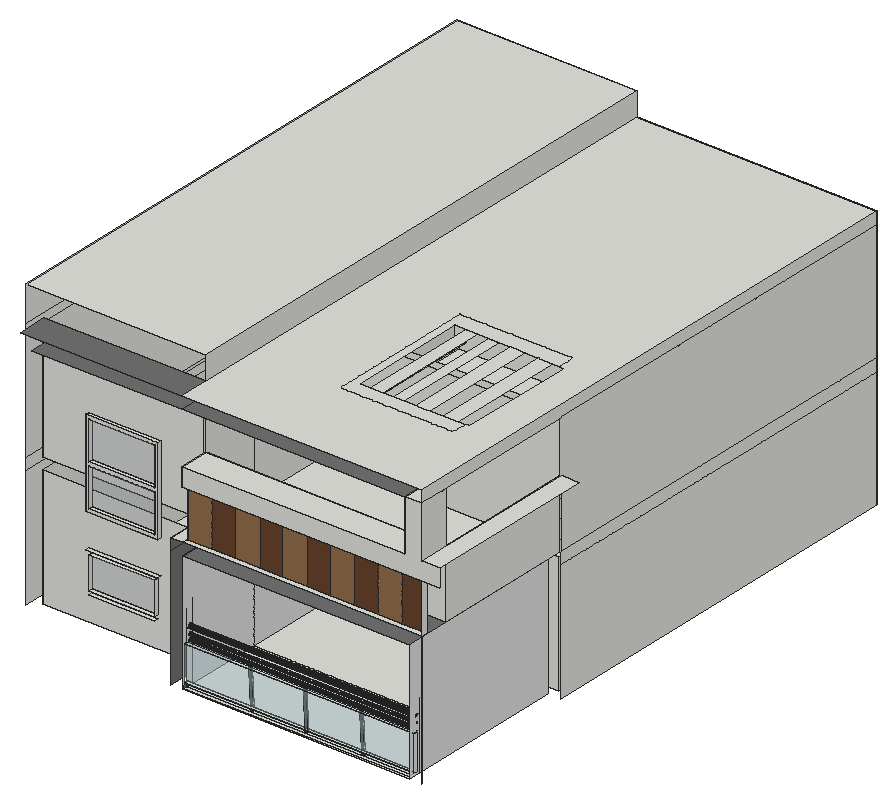
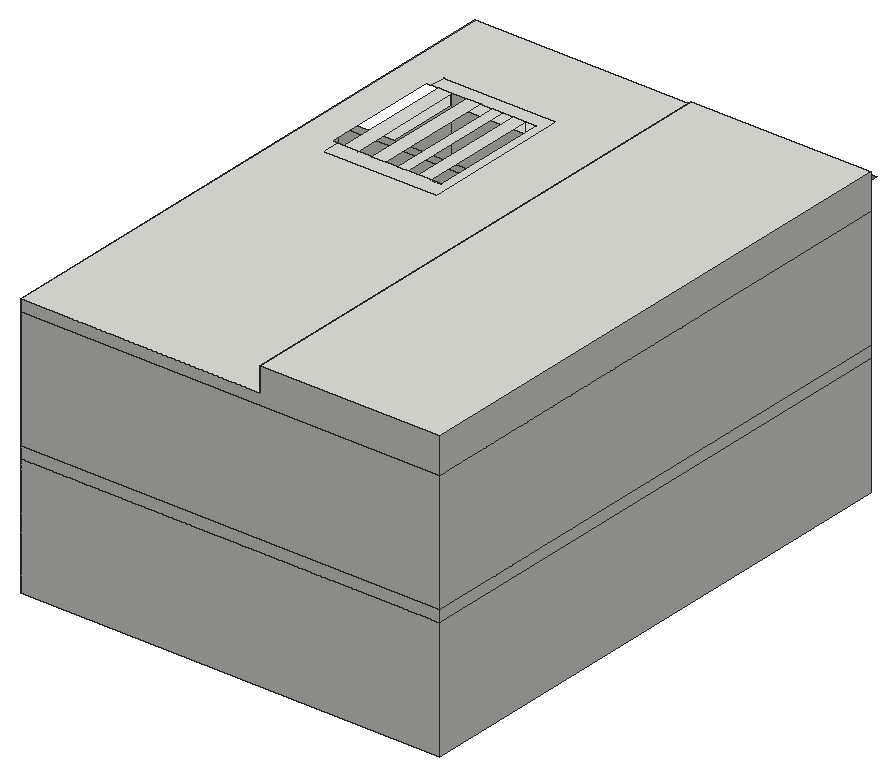
# SketchUp Ruby script. Lengths in inches.
U = 1.inch
M = Sketchup.active_model
def pt(a) = Geom::Point3d.new(a.map { |v| v * U })
def face(e, loops, mat)
  f = e.add_face(loops[0].map { |a| pt(a) })
  loops[1..].each { |l| e.add_face(l.map { |a| pt(a) }).erase! }
  f.material = f.back_material = mat if mat
  f
end
# faces: each face lists its corners as indices into pts; further lists are holes
def faces(e, pts, list, mat = nil) = list.each { |f| face(e, (f[0].is_a?(Array) ? f : [f]).map { |l| l.map { |i| pts[i] } }, mat) }
# xy, xz, yz: faces in a plane at the given z, y or x. An outline is a flat list of corners, or four numbers for a rectangle; further outlines are holes
def ring(l) = l.size == 4 ? [[l[0], l[1]], [l[2], l[1]], [l[2], l[3]], [l[0], l[3]]] : l.each_slice(2).to_a
def flat(e, list, mat, &to3) = list.each { |f| face(e, (f[0].is_a?(Array) ? f : [f]).map { |l| ring(l).map { |u, v| to3.(u, v) } }, mat) }
def xy(e, z, list, mat = nil) = flat(e, list, mat) { |x, y| [x, y, z] }
def xz(e, y, list, mat = nil) = flat(e, list, mat) { |x, z| [x, y, z] }
def yz(e, x, list, mat = nil) = flat(e, list, mat) { |y, z| [x, y, z] }
def lines(e, pts, list) = list.each { |a, b| e.add_line(pt(pts[a]), pt(pts[b])) }
# prism: a flat outline (further loops are holes) pulled along v
def prism(e, loops, v, mat = nil)
  f = face(e, loops, mat); d = Geom::Vector3d.new(v.map { |x| x * U })
  f.pushpull(f.normal.samedirection?(d) ? d.length : -d.length)
end
def box(e, o, s, mat = nil) = prism(e, [[o, [o[0] + s[0], o[1], o[2]], [o[0] + s[0], o[1] + s[1], o[2]], [o[0], o[1] + s[1], o[2]]]], [0, 0, s[2]], mat)
def at(x, y, z, deg = 0) = Geom::Transformation.translation(pt([x, y, z])) * Geom::Transformation.rotation(ORIGIN, Z_AXIS, deg.degrees)
def axes(o, x, y, z) = Geom::Transformation.new([*x, 0, *y, 0, *z, 0, *pt(o).to_a, 1])
def part(name) = M.definitions.add(name)
# library, detail: a bought-in or finely detailed component or shape, given as its bounding box
def library(name, o, s) = part(name).tap { |d| box(d.entities, o, s) }
def detail(e, o, s) = box(e.add_group.entities, o, s)
def put(e, d, t, mat = nil) = e.add_instance(d, t).tap { |i| i.material = mat if mat }
def group(e, t, mat = nil) = e.add_group.tap { |g| g.transformation = t; g.material = mat if mat }.entities
root = M.entities
M.materials.add("Glass_Basic_01").color = [161, 173, 186]
M.materials["Glass_Basic_01"].alpha = 0.25
M.materials.add("Glass_Safety_01").color = [204, 235, 244]
M.materials["Glass_Safety_01"].alpha = 0.25
M.materials.add("M00_Soft_Cloud").color = [255, 255, 255]
M.materials.add("M01_Silver_Fog").color = [224, 224, 224]
M.materials.add("M05_Graphite_Haze").color = [114, 114, 114]
M.materials.add("Metal_06_1K").color = [238, 236, 231]
M.materials.add("Wood_Floor_01_1K").color = [146, 111, 76]
M.materials.add("Wood_Veneer_15_1K").color = [103, 69, 45]
M.materials.add("[Translucent Glass Gray]").color = [132, 132, 132]
M.materials["[Translucent Glass Gray]"].alpha = 0.25
M.materials.add("[Wood Veneer 01]").color = [120, 70, 37]
c1 = part("Group\#8")
xy(c1.entities,0,[[0,0,19.69,1.18]],"[Wood Veneer 01]")
xy(c1.entities,2.76,[[2.76,0,16.93,1.18]],"[Wood Veneer 01]")
xy(c1.entities,60.24,[[2.76,0,16.93,1.18]],"[Wood Veneer 01]")
xy(c1.entities,62.99,[[0,0,19.69,1.18]],"[Wood Veneer 01]")
xz(c1.entities,0,[[2.76,2.76,16.93,60.24]],"[Translucent Glass Gray]")
xz(c1.entities,0,[[[0,0,19.69,62.99],[2.76,2.76,16.93,60.24]]],"[Wood Veneer 01]")
xz(c1.entities,1.18,[[[0,0,19.69,62.99],[2.76,2.76,16.93,60.24]]],"[Wood Veneer 01]")
yz(c1.entities,0,[[0,0,1.18,62.99]],"[Wood Veneer 01]")
yz(c1.entities,2.76,[[0,2.76,1.18,60.24]],"[Wood Veneer 01]")
yz(c1.entities,16.93,[[0,2.76,1.18,60.24]],"[Wood Veneer 01]")
yz(c1.entities,19.69,[[0,0,1.18,62.99]],"[Wood Veneer 01]")
c2 = part("pintu 2")
put(c2.entities,c1,at(-19.69,0,1.97))
g1 = group(c2.entities,at(-21.65,0,0))
prism(g1,[[[0,0,66.93],[0,0,0],[45.28,0,0],[45.28,0,66.93]],[[43.31,0,1.97],[23.62,0,1.97],[23.62,0,64.96],[43.31,0,64.96]],[[21.65,0,64.96],[21.65,0,1.97],[1.97,0,1.97],[1.97,0,64.96]]],[0,5.91,0],"[Wood Veneer 01]")
put(c2.entities,c1,at(1.97,0,1.97))
c3 = library("CLASSIC-BRASS_CHAUTAUQUA_LEVER-HARDWARE",[7.77,-2.58,0],[5.5,6.97,4.76])
xy(root,288,[[271.502,48.443,499.502,49.99],[271.502,49.99,499.502,53.035],[[271.502,53.035,499.502,59.828],[447.56,55.172,447.248,55.213,446.958,55.333,446.709,55.525,446.517,55.774,446.397,56.064,446.356,56.375,446.397,56.687,446.517,56.977,446.709,57.226,446.749,57.258,446.958,57.418,447.248,57.538,447.56,57.579,447.871,57.538,448.161,57.418,448.411,57.226,448.602,56.977,448.722,56.687,448.763,56.375,448.722,56.064,448.602,55.774,448.411,55.525,448.37,55.493,448.161,55.333,447.871,55.213],[334.673,55.172,334.361,55.213,334.071,55.333,333.822,55.525,333.63,55.774,333.51,56.064,333.469,56.375,333.51,56.687,333.63,56.977,333.822,57.226,333.897,57.284,334.071,57.418,334.361,57.538,334.673,57.579,334.984,57.538,335.274,57.418,335.523,57.226,335.715,56.977,335.835,56.687,335.876,56.375,335.835,56.064,335.715,55.774,335.523,55.525,335.448,55.467,335.274,55.333,334.984,55.213],[389.494,55.172,389.183,55.213,388.892,55.333,388.643,55.525,388.452,55.774,388.332,56.064,388.291,56.375,388.332,56.687,388.452,56.977,388.643,57.226,388.719,57.284,388.892,57.418,389.183,57.538,389.494,57.579,389.806,57.538,390.096,57.418,390.345,57.226,390.536,56.977,390.657,56.687,390.698,56.375,390.657,56.064,390.536,55.774,390.345,55.525,390.27,55.467,390.096,55.333,389.806,55.213]],[271.502,59.828,499.502,137.443],[100.502,86.443,262.502,86.443,262.502,230.443,310.876,230.443,310.876,233.831,310.201,233.831,310.201,237.474,307.502,237.474,307.502,238.931,310.876,238.931,310.876,233.831,311.213,233.831,311.213,237.474,364.86,237.474,364.86,238.931,368.234,238.931,368.234,237.474,365.534,237.474,365.534,233.831,364.86,233.831,364.86,230.443,502.502,230.443,502.502,608.443,100.502,608.443],
  [271.502,137.443,499.502,137.443,499.502,221.443,364.86,221.443,364.86,222.901,364.522,222.901,364.522,230.443,311.213,230.443,311.213,222.901,310.876,222.901,310.876,221.443,271.502,221.443],[307.502,221.443,310.876,222.901],[364.86,221.443,367.502,222.901],[367.502,221.443,368.234,222.901],[307.502,222.901,310.876,230.443],
  [310.876,222.901,311.213,230.443],[364.522,222.901,364.86,230.443],[364.86,222.901,367.502,230.443],[310.876,230.443,311.213,230.443,311.213,233.831,310.876,233.831,310.876,237.474,310.201,237.474,310.201,233.831,310.876,233.831],[311.213,230.443,364.522,233.831],
  [364.522,230.443,364.86,231.645],[364.522,231.645,364.86,231.645,364.86,233.831,365.197,233.831,365.197,237.474,364.86,237.474,364.86,233.831,364.522,233.831],[311.213,233.831,364.86,237.474],[365.197,233.831,365.534,237.474],[307.502,237.474,310.876,238.931],
  [364.86,237.474,368.234,238.931]])
xy(root,291.818,[[324.034,233.831,324.709,234.559],[324.034,236.745,324.709,237.474]])
xy(root,293.1875,[[271.502,49.99,502.148,53.035]])
xy(root,306.378,[[410.693,221.443,458.693,230.443]],"M00_Soft_Cloud")
xy(root,322.044,[[157.502,73.443,223.502,77.443]])
xy(root,325.044,[[157.502,73.443,223.502,77.443]])
xy(root,328.294,[[271.502,49.99,502.148,53.035]],"Glass_Safety_01")
xy(root,358.044,[[157.502,73.443,223.502,77.443]])
xy(root,361.044,[[154.502,73.443,226.502,77.443]])
xy(root,366.273,[[324.034,233.831,324.709,234.559],[324.034,236.745,324.709,237.474]])
xy(root,369.9,[[311.213,222.901,364.522,233.831]])
xy(root,370.091,[[310.876,221.443,364.86,222.901],[364.522,222.901,364.86,231.645],[310.201,233.831,310.876,237.474],[310.876,233.831,311.213,237.474],[311.213,233.831,364.86,237.474],
  [364.86,233.831,365.197,237.474],[365.197,233.831,365.534,237.474],[310.876,237.474,364.86,238.931]])
xy(root,371.427,[[310.876,222.901,364.86,237.474]])
xy(root,372,[[307.502,221.443,367.502,222.901],[367.502,221.443,368.234,222.901],[307.502,237.474,368.234,238.931]])
xy(root,372,[[410.693,221.443,458.693,230.443],[307.502,222.901,367.502,230.443]],"M00_Soft_Cloud")
xy(root,395.883,[[154.502,73.443,226.502,77.443]])
xy(root,398.883,[[157.502,73.443,223.502,77.443]])
xy(root,408,[[271.502,48.443,499.502,221.443]],"M05_Graphite_Haze")
xy(root,420,[[259.502,48.443,271.502,77.443],[271.502,48.443,511.502,54.443],[271.502,77.443,511.502,137.443],[271.502,137.443,511.502,221.443]])
xy(root,437.883,[[157.502,73.443,223.502,77.443]])
xy(root,440.883,[[157.502,73.443,223.502,77.443]])
xy(root,470.314,[[271.502,47.443,511.502,54.443]])
xy(root,479.883,[[157.502,73.443,223.502,77.443]])
xy(root,482.883,[[154.502,73.443,226.502,77.443]])
xy(root,488.314,[[271.502,47.443,495.1,77.443],[511.502,47.443,529.502,221.87]])
xy(root,540,[[495.1,47.443,511.502,77.443],[368.076,221.443,378.906,230.443]])
xy(root,540,[[121.502,47.443,271.502,77.443],[271.502,47.443,495.1,77.443]],"M05_Graphite_Haze")
xy(root,552,[[[271.502,47.443,511.502,617.443],[359.302,134.881,359.302,286.083,473.522,286.083,473.522,268.901,478.113,268.901,478.113,150.323,473.522,150.323,473.522,134.881]],[359.302,134.881,473.522,134.881,473.522,150.323,465.869,150.323,465.869,149.955,411.895,149.955,411.895,149.913,401.873,149.913,401.873,150.007,391.136,150.007,391.136,150.048,368.076,150.048,368.076,268.901,473.522,268.901,473.522,286.083,359.302,286.083],[401.873,149.913,411.895,268.901],[424.264,149.955,437.952,268.901],[451.91,149.955,465.869,268.901],
  [378.906,150.048,391.136,268.901]])
xy(root,552,[[109.502,47.443,271.502,77.443]],"M05_Graphite_Haze")
xy(root,576,[[91.502,77.443,271.502,617.443]])
xz(root,47.443,[[271.502,470.314,529.502,470.314,529.502,488.314,511.502,488.314,511.502,540,495.1,540,495.1,488.314,271.502,488.314]])
xz(root,49.99,[[271.502,293.1875,502.148,328.294]],"Glass_Safety_01")
xz(root,53.035,[[271.502,293.1875,502.148,328.294]],"Glass_Safety_01")
xz(root,54.443,[[271.502,420,295.502,470.314],[319.502,420,343.502,470.314],[367.502,420,391.502,470.314],[415.502,420,438.675,470.314],[462.675,420,486.675,470.314]],"Wood_Floor_01_1K")
xz(root,54.443,[[295.502,420,319.502,470.314],[343.502,420,367.502,470.314],[391.502,420,415.502,470.314],[438.675,420,462.675,470.314],[486.675,420,511.502,470.314]],"Wood_Veneer_15_1K")
xz(root,73.443,[[[154.502,395.883,226.502,482.883],[157.502,398.883,223.502,437.883],[157.502,440.883,223.502,479.883]]])
xz(root,77.443,[[271.502,420,271.502,488.314,495.1,488.314,495.1,540,511.502,540,511.502,420]])
xz(root,77.443,[[157.502,325.044,223.502,358.044],[157.502,398.883,223.502,437.883],[157.502,440.883,223.502,479.883]],"Glass_Basic_01")
xz(root,86.443,[[100.502,288,262.502,408],[100.502,420,262.502,540]])
xz(root,221.443,[[307.502,288,310.876,288,310.876,370.091,364.86,370.091,364.86,288,367.502,288,367.502,372,307.502,372],[367.502,288,368.234,372],[271.502,420,511.502,540]])
xz(root,221.443,[[[271.502,288,307.502,288,307.502,372,368.234,372,368.234,288,499.502,288,499.502,408,271.502,408],[410.693,306.378,458.693,372]]],"M00_Soft_Cloud")
xz(root,222.901,[[307.502,288,310.876,370.473],[310.876,288,311.213,370.091],[364.522,288,364.86,370.091],[364.86,288,368.234,370.473],[311.213,369.9,364.522,370.091],
  [310.876,370.091,364.86,371.427],[307.502,370.473,307.502,372,368.234,372,368.234,370.473,364.86,370.473,364.86,371.427,310.876,371.427,310.876,370.473]])
xz(root,230.443,[[[262.502,288,262.502,408,502.502,408,502.502,288,367.502,288,367.502,372,307.502,372,307.502,288],[410.693,306.378,458.693,372]],[262.502,420,502.502,540],[368.076,540,378.906,540.204]])
xz(root,233.831,[[310.201,288,310.876,370.091],[310.876,288,311.213,369.9],[[311.213,288,364.522,369.9],[324.034,291.818,324.709,366.273]],[364.522,288,364.86,369.9],[364.86,288,365.197,370.091],
  [365.197,288,365.534,370.091],[310.876,369.9,311.213,370.091],[311.213,369.9,364.86,370.091]])
xz(root,234.559,[[324.034,291.818,324.709,366.273]])
xz(root,236.745,[[324.034,291.818,324.709,366.273]])
xz(root,237.474,[[307.502,288,310.201,288,310.201,370.091,310.876,370.091,310.876,370.473,307.502,370.473],[310.201,288,310.876,370.091],[[311.213,288,364.86,370.091],[324.034,291.818,324.709,366.273]],[364.86,288,365.197,370.091],[365.534,288,368.234,288,368.234,370.473,364.86,370.473,364.86,370.091,365.534,370.091],
  [365.197,288,365.534,370.091],[310.876,370.091,364.86,371.427],[307.502,370.473,310.876,370.473,310.876,371.427,364.86,371.427,364.86,370.473,368.234,370.473,368.234,372,307.502,372]])
xz(root,238.931,[[307.502,288,307.502,372,368.234,372,368.234,288,364.86,288,364.86,370.091,310.876,370.091,310.876,288]])
xz(root,268.901,[[368.076,540.204,378.906,552]])
xz(root,608.443,[[100.502,288,502.502,408],[100.502,420,502.502,540]])
xz(root,617.443,[[91.502,288,511.502,408],[91.502,408,511.502,420],[91.502,420,511.502,540],[91.502,540,91.502,576,271.502,576,271.502,552,511.502,552,511.502,540]])
yz(root,91.502,[[77.443,288,617.443,408],[77.443,408,617.443,420],[77.443,420,617.443,540],[77.443,540,617.443,576]])
yz(root,100.502,[[86.443,288,608.443,408],[86.443,420,608.443,540]])
yz(root,154.502,[[73.443,395.883,77.443,482.883]])
yz(root,157.502,[[73.443,325.044,77.443,358.044],[73.443,398.883,77.443,437.883],[73.443,440.883,77.443,479.883]])
yz(root,223.502,[[73.443,325.044,77.443,358.044],[73.443,398.883,77.443,437.883],[73.443,440.883,77.443,479.883]])
yz(root,226.502,[[73.443,395.883,77.443,482.883]])
yz(root,259.502,[[48.443,288,77.443,408],[48.443,408,77.443,420]],"M05_Graphite_Haze")
yz(root,262.502,[[86.443,288,137.443,408],[137.443,288,230.443,408],[86.443,420,137.443,540],[137.443,420,230.443,540]])
yz(root,271.502,[[56.49,333.286,56.124,333.335,55.783,333.476,55.49,333.701,55.265,333.994,55.124,334.335,55.075,334.702,55.124,335.068,55.265,335.409,55.49,335.702,55.783,335.927,56.124,336.069,56.49,336.117,56.857,336.069,57.198,335.927,57.491,335.702,57.716,335.409,57.857,335.068,57.906,334.702,57.857,334.335,57.716,333.994,57.491,333.701,57.198,333.476,56.857,333.335],[56.344,339.5,55.812,339.641,55.334,339.914,54.943,340.302,54.666,340.778,54.521,341.309,54.519,341.86,54.66,342.392,54.933,342.87,55.321,343.261,55.797,343.538,56.328,343.683,56.879,343.685,57.411,343.544,57.889,343.271,58.28,342.883,58.557,342.407,58.702,341.876,58.704,341.325,58.563,340.793,58.29,340.315,57.902,339.924,57.426,339.647,56.895,339.503],[54.443,420,60.443,470.314],[60.443,420,77.443,470.314],[77.443,420,137.443,540],
  [137.443,420,221.443,540],[47.443,470.314,77.443,488.314],[77.443,552,617.443,576]])
yz(root,271.502,[[[48.443,288,49.99,288,49.99,328.294,53.035,328.294,53.035,288,137.443,288,137.443,408,48.443,408],[56.344,339.5,55.812,339.641,55.334,339.914,54.943,340.302,54.666,340.778,54.521,341.309,54.519,341.86,54.66,342.392,54.933,342.87,55.321,343.261,55.797,343.538,56.328,343.683,56.879,343.685,57.411,343.544,57.889,343.271,58.28,342.883,58.557,342.407,58.702,341.876,58.704,341.325,58.563,340.793,58.29,340.315,57.902,339.924,57.426,339.647,56.895,339.503],[56.49,333.286,56.124,333.335,55.783,333.476,55.49,333.701,55.265,333.994,55.124,334.335,55.075,334.702,55.124,335.068,55.265,335.409,55.49,335.702,55.783,335.927,56.124,336.069,56.49,336.117,56.857,336.069,57.198,335.927,57.491,335.702,57.716,335.409,57.857,335.068,57.906,334.702,57.857,334.335,57.716,333.994,57.491,333.701,57.198,333.476,56.857,333.335]],[137.443,288,221.443,408]],"M01_Silver_Fog")
yz(root,271.502,[[49.99,288,53.035,293.1875]],"M05_Graphite_Haze")
yz(root,307.502,[[221.443,288,222.901,372],[237.474,288,238.931,372]])
yz(root,307.502,[[222.901,288,230.443,372]],"M00_Soft_Cloud")
yz(root,310.201,[[233.831,288,237.474,370.091]])
yz(root,310.876,[[221.443,288,222.901,370.091],[222.901,288,222.901,371.427,237.474,371.427,237.474,370.091,233.831,370.091,233.831,288],[233.831,288,237.474,369.9],[237.474,288,238.931,370.091],[233.831,369.9,237.474,370.091]])
yz(root,311.213,[[222.901,288,233.831,369.9],[233.831,288,237.474,370.091]])
yz(root,324.034,[[233.831,291.818,234.559,366.273],[236.745,291.818,237.474,366.273]])
yz(root,324.709,[[233.831,291.818,234.559,366.273],[236.745,291.818,237.474,366.273]])
yz(root,364.522,[[222.901,288,233.831,369.9],[222.901,369.9,231.645,370.091]])
yz(root,364.86,[[221.443,288,222.901,370.091],[222.901,288,231.645,370.091],[231.645,288,233.831,288,233.831,370.091,237.474,370.091,237.474,371.427,222.901,371.427,222.901,370.091,231.645,370.091],[233.831,288,237.474,369.9],[237.474,288,238.931,370.091],
  [233.831,369.9,237.474,370.091]])
yz(root,365.197,[[233.831,288,237.474,370.091]])
yz(root,365.534,[[233.831,288,237.474,370.091]])
yz(root,367.502,[[221.443,288,230.443,372]],"M00_Soft_Cloud")
yz(root,368.234,[[221.443,288,222.901,372],[237.474,288,238.931,372]])
yz(root,410.693,[[221.443,306.378,230.443,372]],"M00_Soft_Cloud")
yz(root,458.693,[[221.443,306.378,230.443,372]],"M00_Soft_Cloud")
yz(root,495.1,[[47.443,488.314,77.443,540]])
yz(root,499.502,[[[48.443,288,221.443,408],[56.344,339.5,56.895,339.503,57.426,339.647,57.902,339.924,58.29,340.315,58.563,340.793,58.704,341.325,58.702,341.876,58.557,342.407,58.28,342.883,57.889,343.271,57.411,343.544,56.879,343.685,56.328,343.683,55.797,343.538,55.321,343.261,54.933,342.87,54.66,342.392,54.519,341.86,54.521,341.309,54.666,340.778,54.943,340.302,55.334,339.914,55.812,339.641],[56.49,333.286,56.857,333.335,57.198,333.476,57.491,333.701,57.716,333.994,57.857,334.335,57.906,334.702,57.857,335.068,57.716,335.409,57.491,335.702,57.198,335.927,56.857,336.069,56.49,336.117,56.124,336.069,55.783,335.927,55.49,335.702,55.265,335.409,55.124,335.068,55.075,334.702,55.124,334.335,55.265,333.994,55.49,333.701,55.783,333.476,56.124,333.335],[56.895,323.269,57.261,323.317,57.602,323.458,57.896,323.683,58.12,323.976,58.262,324.318,58.31,324.684,58.262,325.05,58.12,325.391,57.896,325.684,57.602,325.909,57.261,326.051,56.895,326.099,56.529,326.051,56.187,325.909,55.894,325.684,55.669,325.391,55.528,325.05,55.48,324.684,55.528,324.318,55.669,323.976,55.894,323.683,56.187,323.458,56.529,323.317]]],"M01_Silver_Fog")
yz(root,502.148,[[49.99,293.1875,53.035,328.294]])
yz(root,502.502,[[230.443,288,608.443,408],[230.443,420,608.443,540]])
yz(root,511.502,[[47.443,288,48.443,408],[221.87,288,617.443,408],[47.443,408,48.443,420],[221.87,408,617.443,420],[47.443,420,54.443,470.314],
  [77.443,420,221.443,488.314],[221.443,420,221.87,488.314],[221.87,420,617.443,420,617.443,540,221.443,540,221.443,488.314,221.87,488.314],[47.443,488.314,77.443,540],[47.443,540,617.443,552]])
p = [[332.916,54.348,328.331],[334.071,55.333,288],[334.361,55.213,288],[333.207,54.228,328.336],[334.673,55.172,288],[333.518,54.187,328.344],
  [334.984,55.213,288],[333.829,54.228,328.354],[335.274,55.333,288],[334.119,54.348,328.365],[444.16,54.348,328.331],[445.314,55.333,288],
  [445.604,55.213,288],[444.45,54.228,328.336],[445.916,55.172,288],[444.761,54.187,328.344],[446.227,55.213,288],[445.072,54.228,328.354],
  [446.517,55.333,288],[445.362,54.348,328.365],[332.667,54.54,328.329],[333.822,55.525,288],[335.448,55.467,288],[335.523,55.524,288.004],
  [334.368,54.539,328.377],[389.183,55.213,288],[388.121,54.307,325.107],[387.831,54.427,325.101],[388.892,55.333,288],[389.494,55.172,288],
  [388.432,54.266,325.115],[389.806,55.213,288],[388.743,54.307,325.124],[390.096,55.333,288],[389.033,54.427,325.136],[443.911,54.54,328.329],
  [445.065,55.525,288],[446.691,55.467,288],[446.767,55.524,288.004],[445.611,54.539,328.377],[387.581,54.619,325.099],[388.643,55.525,288],
  [390.345,55.524,288.004],[389.282,54.617,325.147],[390.27,55.467,288],[332.476,54.789,328.329],[333.63,55.774,288],[335.714,55.773,288.015],
  [334.559,54.788,328.389],[443.719,54.789,328.329],[444.874,55.774,288],[446.958,55.773,288.015],[445.802,54.788,328.389],[387.39,54.868,325.099],
  [388.452,55.774,288],[389.473,54.866,325.159],[390.536,55.773,288.015],[332.356,55.079,328.333],[333.51,56.064,288],[335.834,56.063,288.026],
  [334.679,55.078,328.399],[443.599,55.079,328.333],[444.753,56.064,288],[447.077,56.063,288.026],[445.922,55.078,328.399],[387.27,55.158,325.103],
  [388.332,56.064,288],[389.593,55.156,325.17],[390.656,56.063,288.026],[332.315,55.39,328.339],[333.469,56.375,288],[335.875,56.375,288.034],
  [334.719,55.389,328.408],[443.558,55.39,328.339],[444.712,56.375,288],[447.118,56.375,288.034],[445.963,55.389,328.408],[335.834,56.686,288.041],
  [335.713,56.976,288.044],[335.522,57.225,288.045],[335.273,57.417,288.043],[334.983,57.537,288.037],[334.672,57.578,288.029],[334.361,57.537,288.019],
  [334.071,57.417,288.008],[333.897,57.284,288],[333.822,57.227,287.996],[333.631,56.978,287.985],[333.511,56.6875,287.974],[333.47,56.376,287.966],
  [333.511,56.065,287.959],[333.632,55.775,287.956],[333.823,55.526,287.955],[334.072,55.334,287.957],[334.362,55.214,287.963],[334.673,55.173,287.971],
  [334.985,55.214,287.981],[335.274,55.333,287.992],[387.229,55.469,325.11],[388.291,56.375,288],[388.892,55.334,287.976],[388.643,55.525,287.98],
  [388.452,55.774,287.986],[388.332,56.064,287.993],[388.332,56.687,288.007],[388.452,56.977,288.014],[388.643,57.226,288.02],[388.892,57.417,288.024],
  [389.183,57.537,288.027],[389.449,57.572,288.028],[389.494,57.578,288.028],[389.806,57.537,288.027],[390.096,57.417,288.024],[390.345,57.226,288.02],
  [390.536,56.977,288.014],[390.657,56.687,288.007],[390.698,56.375,288],[390.657,56.064,287.993],[390.536,55.774,287.986],[390.345,55.525,287.98],
  [390.096,55.334,287.976],[389.806,55.214,287.973],[389.494,55.173,287.972],[389.183,55.214,287.973],[389.633,55.468,325.178],[390.697,56.375,288.034],
  [448.721,56.686,288.031],[448.601,56.977,288.034],[448.41,57.226,288.035],[448.161,57.417,288.033],[447.871,57.537,288.029],[447.559,57.578,288.024],
  [447.248,57.538,288.016],[446.958,57.418,288.008],[446.749,57.258,288],[446.709,57.226,287.999],[446.518,56.977,287.99],[446.398,56.6875,287.981],
  [446.357,56.376,287.974],[446.398,56.065,287.969],[446.518,55.774,287.966],[446.709,55.525,287.965],[446.959,55.334,287.967],[447.249,55.214,287.971],
  [447.56,55.173,287.976],[447.871,55.213,287.984],[448.162,55.333,287.992],[448.37,55.493,288],[448.411,55.524,288.001],[448.602,55.774,288.01],
  [448.722,56.064,288.019],[448.763,56.375,288.026],[447.248,55.213,288],[446.958,55.333,288],[447.56,55.172,288],[447.871,55.213,288],
  [448.161,55.333,288],[390.345,55.525,288],[446.709,55.525,288],[332.355,55.702,328.348],[333.51,56.687,288],[334.678,55.7,328.414],
  [443.598,55.702,328.348],[444.753,56.687,288],[447.077,56.686,288.041],[445.921,55.7,328.414],[387.269,55.781,325.118],[388.332,56.687,288],
  [389.592,55.779,325.185],[390.655,56.686,288.041],[390.536,55.774,288],[446.517,55.774,288],[332.475,55.992,328.358],[333.63,56.977,288],
  [334.558,55.99,328.418],[443.718,55.992,328.358],[444.874,56.977,288],[446.957,56.976,288.044],[445.801,55.99,328.418],[387.389,56.071,325.129],
  [388.452,56.977,288],[389.472,56.069,325.188],[390.535,56.976,288.044],[390.657,56.064,288],[446.397,56.064,288],[332.666,56.241,328.37],
  [333.822,57.226,288],[334.367,56.239,328.419],[443.909,56.241,328.37],[445.065,57.226,288],[446.765,57.225,288.045],[445.61,56.239,328.419],
  [387.58,56.32,325.14],[388.643,57.226,288],[389.281,56.318,325.189],[390.344,57.225,288.045],[446.356,56.375,288],[332.915,56.432,328.382],
  [334.117,56.431,328.416],[445.314,57.417,288.008],[445.14,57.284,288],[444.158,56.432,328.382],[446.516,57.417,288.043],[445.361,56.431,328.416],
  [387.829,56.511,325.152],[388.892,57.417,288.008],[388.719,57.284,288],[389.032,56.51,325.187],[390.095,57.417,288.043],[333.205,56.552,328.393],
  [333.827,56.551,328.411],[445.604,57.537,288.019],[444.448,56.552,328.393],[446.226,57.537,288.037],[445.071,56.551,328.411],[446.397,56.687,288],
  [388.119,56.63,325.163],[389.182,57.537,288.019],[388.741,56.63,325.181],[389.805,57.537,288.037],[333.516,56.592,328.403],[389.493,57.578,288.029],
  [388.43,56.671,325.173],[445.915,57.578,288.029],[444.759,56.592,328.403],[446.517,56.977,288],[446.709,57.226,288],[387.738,54.348,328.331],
  [388.028,54.228,328.336],[388.339,54.187,328.344],[388.651,54.228,328.354],[388.941,54.348,328.365],[387.489,54.54,328.329],[389.189,54.539,328.377],
  [387.298,54.789,328.329],[389.38,54.788,328.389],[387.177,55.079,328.333],[387.136,55.39,328.339],[387.177,55.702,328.348],[387.297,55.992,328.358],
  [387.488,56.241,328.37],[387.737,56.432,328.382],[389.5,55.078,328.399],[389.541,55.389,328.408],[389.5,55.7,328.414],[389.38,55.99,328.418],
  [389.188,56.239,328.419],[388.939,56.431,328.416],[388.027,56.552,328.393],[388.649,56.551,328.411],[388.338,56.592,328.403],[271.502,56.529,327.574],
  [271.502,56.895,327.526],[499.502,56.895,327.526],[499.502,56.529,327.574],[271.502,57.261,327.574],[499.502,57.261,327.574],[271.502,56.187,327.716],
  [499.502,56.187,327.716],[271.502,57.602,327.716],[499.502,57.602,327.716],[271.502,55.894,327.941],[499.502,55.894,327.941],[271.502,57.896,327.941],
  [499.502,57.896,327.941],[271.502,55.669,328.234],[499.502,55.669,328.234],[447.995,55.669,328.234],[446.791,55.669,328.234],[271.502,58.12,328.234],
  [499.502,58.12,328.234],[271.502,55.528,328.575],[499.502,55.528,328.575],[390.698,55.528,328.575],[389.494,55.528,328.575],[388.291,55.528,328.575],
  [271.502,58.262,328.575],[499.502,58.262,328.575],[271.502,55.48,328.941],[499.502,55.48,328.941],[334.826,55.48,328.941],[333.623,55.48,328.941],
  [271.502,58.31,328.941],[499.502,58.31,328.941],[271.502,55.528,329.307],[499.502,55.528,329.307],[271.502,58.262,329.307],[499.502,58.262,329.307],
  [271.502,55.669,329.649],[499.502,55.669,329.649],[271.502,58.12,329.649],[499.502,58.12,329.649],[271.502,55.894,329.942],[499.502,55.894,329.942],
  [271.502,57.896,329.942],[499.502,57.896,329.942],[271.502,56.187,330.167],[499.502,56.187,330.167],[271.502,57.602,330.167],[499.502,57.602,330.167],
  [271.502,56.529,330.308],[499.502,56.529,330.308],[271.502,57.261,330.308],[499.502,57.261,330.308],[271.502,56.895,330.356],[499.502,56.895,330.356],
  [271.502,55.783,333.476],[271.502,56.124,333.335],[499.502,56.124,333.335],[499.502,55.783,333.476],[271.502,56.49,333.286],[499.502,56.49,333.286],
  [271.502,56.857,333.335],[499.502,56.857,333.335],[271.502,57.198,333.476],[499.502,57.198,333.476],[271.502,55.49,333.701],[499.502,55.49,333.701],
  [271.502,57.491,333.701],[499.502,57.491,333.701],[271.502,55.265,333.994],[499.502,55.265,333.994],[271.502,57.716,333.994],[499.502,57.716,333.994],
  [271.502,55.124,334.335],[499.502,55.124,334.335],[271.502,57.857,334.335],[499.502,57.857,334.335],[271.502,55.075,334.702],[499.502,55.075,334.702],
  [271.502,57.906,334.702],[499.502,57.906,334.702],[271.502,55.124,335.068],[499.502,55.124,335.068],[271.502,57.857,335.068],[499.502,57.857,335.068],
  [271.502,55.265,335.409],[499.502,55.265,335.409],[271.502,57.716,335.409],[499.502,57.716,335.409],[271.502,55.49,335.702],[499.502,55.49,335.702],
  [271.502,57.491,335.702],[499.502,57.491,335.702],[271.502,55.783,335.927],[499.502,55.783,335.927],[271.502,57.198,335.927],[499.502,57.198,335.927],
  [271.502,56.124,336.069],[499.502,56.124,336.069],[271.502,56.857,336.069],[499.502,56.857,336.069],[271.502,56.49,336.117],[499.502,56.49,336.117],
  [271.502,55.812,339.641],[271.502,56.344,339.5],[499.502,56.344,339.5],[499.502,55.812,339.641],[271.502,56.895,339.503],[499.502,56.895,339.503],
  [271.502,57.426,339.647],[499.502,57.426,339.647],[271.502,55.334,339.914],[499.502,55.334,339.914],[271.502,57.902,339.924],[499.502,57.902,339.924],
  [271.502,54.943,340.302],[499.502,54.943,340.302],[271.502,58.29,340.315],[499.502,58.29,340.315],[271.502,54.666,340.778],[499.502,54.666,340.778],
  [271.502,58.563,340.793],[499.502,58.563,340.793],[271.502,54.521,341.309],[499.502,54.521,341.309],[271.502,58.704,341.325],[499.502,58.704,341.325],
  [271.502,54.519,341.86],[499.502,54.519,341.86],[271.502,58.702,341.876],[499.502,58.702,341.876],[271.502,54.66,342.392],[499.502,54.66,342.392],
  [271.502,58.557,342.407],[499.502,58.557,342.407],[271.502,54.933,342.87],[499.502,54.933,342.87],[271.502,58.28,342.883],[499.502,58.28,342.883],
  [271.502,55.321,343.261],[499.502,55.321,343.261],[271.502,57.889,343.271],[499.502,57.889,343.271],[271.502,55.797,343.538],[499.502,55.797,343.538],
  [271.502,57.411,343.544],[499.502,57.411,343.544],[271.502,56.328,343.683],[499.502,56.328,343.683],[271.502,56.879,343.685],[499.502,56.879,343.685],
  [271.502,56.611,341.593],[499.502,56.611,341.593],[271.502,56.895,333.813],[499.502,56.895,333.813],[499.502,59.828,355.815],[499.502,59.828,288],
  [271.502,59.828,288],[271.502,59.828,365.773],[388.643,54.677,324.298],[388.452,54.927,324.304],[388.332,55.217,324.31],[388.291,55.528,324.318],
  [388.332,55.839,324.325],[388.452,56.129,324.332],[388.892,56.57,324.342],[389.183,56.69,324.345],[389.494,56.731,324.346],[389.806,56.69,324.345],
  [390.096,56.57,324.342],[390.345,56.378,324.337],[390.536,56.129,324.332],[390.657,55.839,324.325],[390.698,55.528,324.318],[390.657,55.217,324.31],
  [390.536,54.927,324.304],[390.345,54.677,324.298],[390.096,54.486,324.293],[389.806,54.366,324.29],[389.494,54.325,324.289],[447.953,55.98,324.007],
  [447.994,55.669,324.002],[447.953,55.357,323.995],[447.833,55.067,323.987],[447.642,54.818,323.978],[447.393,54.627,323.969],[447.103,54.507,323.96],
  [446.792,54.466,323.953],[446.48,54.507,323.947],[445.75,55.068,323.942],[445.629,55.358,323.945],[445.588,55.67,323.951],[445.629,55.981,323.958],
  [446.189,56.711,323.984],[446.479,56.831,323.992],[446.791,56.872,324],[447.102,56.831,324.006],[447.392,56.711,324.01],[447.641,56.52,324.011],
  [447.833,56.27,324.01],[389.183,54.366,324.29],[334.673,56.375,288],[333.623,55.48,324.684],[389.275,55.292,284.77],[388.985,55.412,284.77],
  [390.362,55.545,284.77],[390.188,55.412,284.77],[389.898,55.292,284.77],[389.587,55.251,284.77],[388.736,55.603,284.77],[388.544,55.853,284.77],
  [388.424,56.143,284.77],[388.383,56.454,284.77],[388.424,56.766,284.77],[388.544,57.056,284.77],[388.736,57.305,284.77],[388.811,57.363,284.77],
  [390.4375,55.603,284.774],[390.789,56.453,284.805],[390.748,56.765,284.811],[390.628,55.852,284.785],[390.748,56.142,284.796],[389.897,57.616,284.808],
  [389.586,57.657,284.8],[389.275,57.616,284.79],[388.985,57.496,284.779],[390.436,57.304,284.815],[390.187,57.495,284.813],[390.628,57.055,284.815],
  [271.502,53.035,328.294],[271.502,53.035,358.797],[368.076,150.048,540],[378.906,150.048,540],[378.906,150.048,552],[368.076,150.048,552],
  [378.906,221.443,540],[368.076,221.443,540],[368.076,268.901,540.204],[368.076,230.443,540.204],[378.906,268.901,540.204],[378.906,230.443,540.204]]
faces(root,p,[[0,1,2,3],[3,2,4,5],[5,4,6,7],[7,6,8,9],[10,11,12,13],[13,12,14,15],[15,14,16,17],[17,16,18,19],
  [20,21,1,0],[9,8,22,23,24],[25,26,27,28],[29,30,26,25],[31,32,30,29],[33,34,32,31],[35,36,11,10],[19,18,37,38,39],
  [28,27,40,41],[42,43,34,33,44],[45,46,21,20],[47,23,24,48],[49,50,36,35],[51,38,39,52],[41,40,53,54],[42,43,55,56],
  [57,58,46,45],[59,47,48,60],[61,62,50,49],[63,51,52,64],[54,53,65,66],[56,55,67,68],[69,70,58,57],[71,59,60,72],
  [73,74,62,61],[75,63,64,76],[66,65,98,99],[68,67,124,125],[159,160,70,69],[77,71,72,161],[162,163,74,73],[164,75,76,165],
  [99,98,166,104,167],[125,124,168,169],[172,173,160,159],[78,77,161,174],[175,176,163,162],[177,164,165,178],[104,166,179,105,180,167],[169,168,181,182],
  [185,186,173,172],[79,78,174,187],[188,189,176,175],[190,177,178,191],[105,179,192,106,193,180],[182,181,194,195],[84,85,186,185,197],[80,79,187,198],
  [199,200,189,188,201],[202,190,191,203],[106,192,204,107,205,206,193],[195,194,207,208],[84,83,209,197],[81,80,198,210],[199,211,212,201],[213,202,203,214],
  [108,216,204,107,205,217],[208,207,218,219],[83,82,220,209],[82,81,210,220],[221,222,216,108,217,109],[219,218,222,221],[211,223,224,212],[223,213,214,224],
  [227,27,26,228],[228,26,30,229],[229,30,32,230],[230,32,34,231],[232,40,27,227],[231,34,43,233],[234,53,40,232],[235,55,43,233],
  [236,65,53,234],[237,98,65,236],[238,166,98,237],[239,179,166,238],[240,192,179,239],[241,204,192,240],[242,67,55,235],[243,124,67,242],
  [244,168,124,243],[245,181,168,244],[246,194,181,245],[247,207,194,246],[241,204,216,248],[249,218,207,247],[248,216,222,250],[250,222,218,249],
  [251,252,253,254],[252,255,256,253],[257,251,254,258],[255,259,260,256],[261,257,258,262],[259,263,264,260],[265,261,262,266,267,268],[263,269,270,264],
  [271,265,268,267,266,272,273,274,275],[269,276,277,270],[278,271,275,274,273,272,279,280,281],[276,282,283,277],[284,278,281,280,279,285],[282,286,287,283],[288,284,285,289],[286,290,291,287],
  [292,288,289,293],[290,294,295,291],[296,292,293,297],[294,298,299,295],[300,296,297,301],[298,302,303,299],[304,300,301,305],[302,304,305,303],
  [306,307,308,309],[307,310,311,308],[310,312,313,311],[312,314,315,313],[316,306,309,317],[314,318,319,315],[320,316,317,321],[318,322,323,319],
  [324,320,321,325],[322,326,327,323],[328,324,325,329],[326,330,331,327],[332,328,329,333],[330,334,335,331],[336,332,333,337],[334,338,339,335],
  [340,336,337,341],[338,342,343,339],[344,340,341,345],[342,346,347,343],[348,344,345,349],[346,350,351,347],[352,348,349,353],[350,352,353,351],
  [354,355,356,357],[355,358,359,356],[358,360,361,359],[362,354,357,363],[360,364,365,361],[366,362,363,367],[364,368,369,365],[370,366,367,371],
  [368,372,373,369],[374,370,371,375],[372,376,377,373],[378,374,375,379],[376,380,381,377],[382,378,379,383],[380,384,385,381],[386,382,383,387],
  [384,388,389,385],[390,386,387,391],[388,392,393,389],[394,390,391,395],[392,396,397,393],[398,394,395,399],[396,400,401,397],[400,398,399,401]],"Metal_06_1K")
faces(root,p,[[77,78,79,80,81,82,83,84,85,86,87,88,89,90,91,92,93,94,95,96,97,22,23,47,59,71],[2,94,93,1],[4,95,94,2],[6,96,95,4],[8,97,96,6],[100,101,102,103,99,104,105,106,107,108,109,110,111,112,113,114,115,116,117,118,119,120,121,122,123],[123,25,28,100],[122,29,25,123],
  [121,31,29,122],[120,33,31,121],[126,127,128,129,130,131,132,133,134,135,136,137,138,139,140,141,142,143,144,145,146,147,148,149,150,151],[152,143,142,153],[154,144,143,152],[155,145,144,154],[156,146,145,155],[1,93,92,21],
  [22,97,8],[100,28,41,101],[119,157,44,33,120],[153,142,141,158],[147,146,156],[21,92,91,46],[101,41,54,102],[118,170,157,119],
  [158,141,140,171],[46,91,90,58],[102,54,66,103],[117,183,170,118],[171,140,139,184],[58,90,89,70],[103,66,99],[117,116,183],
  [184,139,138,196],[70,89,88,160],[196,138,137,215],[160,88,87,173],[215,137,136,225],[173,87,86,186],[225,136,135,226],[186,86,85],
  [226,135,134],[174,161,72,60,48,24,9,7,5,3,0,20,45,57,69,159,172,185,197,209,220,210,198,187]])
lines(root,p,[[402,403],[404,405],[406,407],[408,409],[410,411],[411,412],[412,413],[413,414],[414,415],[416,417],[417,418],[418,419],
  [419,420],[420,421],[421,422],[422,423],[423,424],[424,425],[425,426],[426,427],[427,428],[428,429],[429,430],[431,432],
  [432,433],[433,434],[434,435],[435,436],[436,437],[437,438],[438,439],[440,441],[441,442],[442,443],[444,445],[445,446],
  [446,447],[447,448],[448,449],[449,450],[450,431],[430,451],[452,453],[454,455],[456,457],[457,458],[458,459],[459,454],
  [455,460],[460,461],[461,462],[462,463],[463,464],[464,465],[465,466],[466,467],[456,468],[469,470],[471,472],[468,471],
  [472,469],[473,474],[474,475],[475,476],[477,478],[476,467],[478,473],[470,479],[479,477],[480,481],[482,483],[484,483],
  [485,482],[486,483],[487,482],[488,489],[490,491]])
put(root,c2,axes([433.65,221.44,306.38],[1.06017,0,0],[0,1,0],[0,0,0.98046]))
put(root,c3,axes([336.84,237.33,324.3],[-1.71399,0,0],[0,-1.8508,0],[0,0,-0.96982]))
